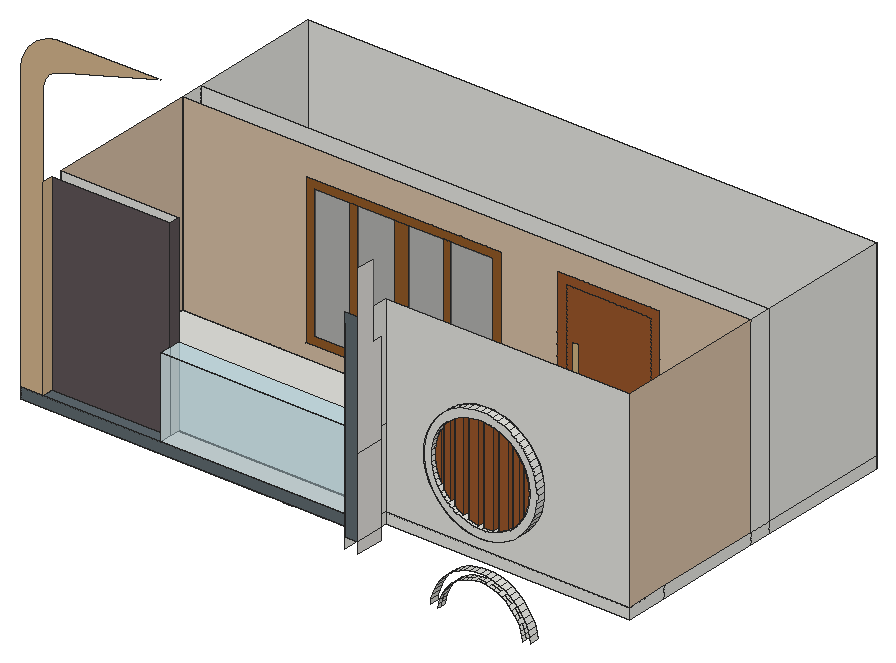
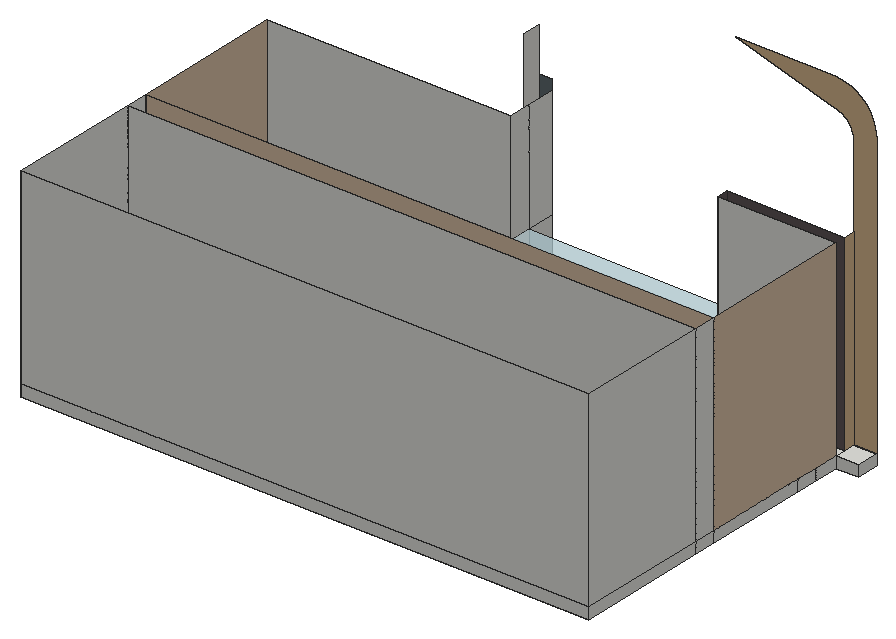
# SketchUp Ruby script. Lengths in inches.
U = 1.inch
M = Sketchup.active_model
def pt(a) = Geom::Point3d.new(a.map { |v| v * U })
def face(e, loops, mat)
  f = e.add_face(loops[0].map { |a| pt(a) })
  loops[1..].each { |l| e.add_face(l.map { |a| pt(a) }).erase! }
  f.material = f.back_material = mat if mat
  f
end
# faces: each face lists its corners as indices into pts; further lists are holes
def faces(e, pts, list, mat = nil) = list.each { |f| face(e, (f[0].is_a?(Array) ? f : [f]).map { |l| l.map { |i| pts[i] } }, mat) }
# xy, xz, yz: faces in a plane at the given z, y or x. An outline is a flat list of corners, or four numbers for a rectangle; further outlines are holes
def ring(l) = l.size == 4 ? [[l[0], l[1]], [l[2], l[1]], [l[2], l[3]], [l[0], l[3]]] : l.each_slice(2).to_a
def flat(e, list, mat, &to3) = list.each { |f| face(e, (f[0].is_a?(Array) ? f : [f]).map { |l| ring(l).map { |u, v| to3.(u, v) } }, mat) }
def xy(e, z, list, mat = nil) = flat(e, list, mat) { |x, y| [x, y, z] }
def xz(e, y, list, mat = nil) = flat(e, list, mat) { |x, z| [x, y, z] }
def yz(e, x, list, mat = nil) = flat(e, list, mat) { |y, z| [x, y, z] }
def lines(e, pts, list) = list.each { |a, b| e.add_line(pt(pts[a]), pt(pts[b])) }
# prism: a flat outline (further loops are holes) pulled along v
def prism(e, loops, v, mat = nil)
  f = face(e, loops, mat); d = Geom::Vector3d.new(v.map { |x| x * U })
  f.pushpull(f.normal.samedirection?(d) ? d.length : -d.length)
end
def box(e, o, s, mat = nil) = prism(e, [[o, [o[0] + s[0], o[1], o[2]], [o[0] + s[0], o[1] + s[1], o[2]], [o[0], o[1] + s[1], o[2]]]], [0, 0, s[2]], mat)
def at(x, y, z, deg = 0) = Geom::Transformation.translation(pt([x, y, z])) * Geom::Transformation.rotation(ORIGIN, Z_AXIS, deg.degrees)
def axes(o, x, y, z) = Geom::Transformation.new([*x, 0, *y, 0, *z, 0, *pt(o).to_a, 1])
def part(name) = M.definitions.add(name)
# library, detail: a bought-in or finely detailed component or shape, given as its bounding box
def library(name, o, s) = part(name).tap { |d| box(d.entities, o, s) }
def detail(e, o, s) = box(e.add_group.entities, o, s)
def put(e, d, t, mat = nil) = e.add_instance(d, t).tap { |i| i.material = mat if mat }
def group(e, t, mat = nil) = e.add_group.tap { |g| g.transformation = t; g.material = mat if mat }.entities
root = M.entities
M.materials.add("[0035_Tan]").color = [210, 180, 140]
M.materials.add("[Asphalt New]").color = [94, 84, 87]
M.materials.add("[Formica Laminate Dark]").color = [50, 53, 60]
M.materials.add("[Formica Laminate Light]").color = [213, 189, 164]
M.materials.add("[Formica Speckled Grey]1").color = [94, 105, 111]
M.materials.add("[Terrazzo Tile Accent]").color = [224, 221, 217]
M.materials.add("[Translucent Glass Gray]").color = [128, 128, 128]
M.materials["[Translucent Glass Gray]"].alpha = 0.5
M.materials.add("[Translucent Glass Safety]").color = [204, 235, 244]
M.materials["[Translucent Glass Safety]"].alpha = 0.5
M.materials.add("[Wood Cherry Original]").color = [152, 86, 42]
M.materials.add("[Wood Floor Light]").color = [204, 176, 127]
M.materials.add("[Wood Floor Parquet]").color = [145, 89, 39]
xy(root,318.5,[[192.74,22.75,199.15,40.6875],[201.68,22.75,208.09,40.6875],[210.74,22.75,217.15,40.6875],[219.8,22.75,226.21,40.6875],[228.49,22.75,234.9,40.6875],
  [237.55,22.75,243.96,40.6875],[246.43,22.75,252.84,40.6875],[255.74,22.75,262.15,40.6875],[264.27,22.75,277.85,40.6875],[264.27,40.6875,277.85,49.71],
  [17.9375,61.15,34.45,78.66],[17.9375,162.27,472.4375,180.28],[17.9375,180.28,472.4375,287.24]])
xy(root,318.5,[[0,22.75,192.74,22.75,192.74,49.71,199.15,49.71,199.15,22.75,201.68,22.75,201.68,49.71,208.09,49.71,208.09,22.75,210.74,22.75,210.74,49.71,217.15,49.71,217.15,22.75,219.8,22.75,219.8,49.71,226.21,49.71,226.21,22.75,228.49,22.75,228.49,49.71,234.9,49.71,234.9,22.75,237.55,22.75,237.55,49.71,243.96,49.71,243.96,22.75,246.43,22.75,246.43,49.71,252.84,49.71,252.84,22.75,255.74,22.75,255.74,49.71,262.15,49.71,262.15,22.75,264.27,22.75,264.27,49.71,277.85,49.71,277.85,40.6875,472.4375,40.6875,472.4375,162.27,17.9375,162.27,17.9375,78.66,34.45,78.66,34.45,61.15,17.9375,61.15,17.9375,40.6875,0,40.6875]],"[Formica Speckled Grey]1")
xy(root,327.375,[[0,22.75,17.9375,40.6875],[112.18,22.75,277.85,40.6875],[17.9375,31.75,112.18,40.6875],[17.9375,40.6875,472.4375,162.27],[17.9375,162.27,472.4375,180.28],
  [17.9375,180.28,472.4375,287.24]])
xy(root,327.375,[[17.9375,22.75,112.18,31.75]],"[Formica Speckled Grey]1")
xy(root,390.5625,[[112.18,22.75,277.85,40.6875]],"[Translucent Glass Safety]")
xz(root,0,[[277.85,327.375,288.19,488.3125]],"[Formica Speckled Grey]1")
xz(root,15.8125,[[[373.3125,352.86,378.06,353.11,382.75,353.85,387.33,355.08,391.77,356.78,396,358.9375,399.98,361.53,403.67,364.51,407.03,367.87,410.02,371.5625,412.61,375.55,414.76,379.78,416.47,384.21,417.7,388.8,418.4375,393.49,418.6875,398.23,418.4375,402.98,417.7,407.67,416.47,412.26,414.76,416.69,412.61,420.92,410.02,424.91,407.03,428.6,403.67,431.95,399.98,434.94,396,437.53,391.77,439.6875,387.33,441.39,382.75,442.62,378.06,443.36,373.3125,443.61,368.57,443.36,363.88,442.62,359.29,441.39,354.86,439.6875,350.625,437.53,346.64,434.94,342.95,431.95,339.59,428.6,336.6,424.91,334.02,420.92,331.86,416.69,330.16,412.26,328.93,407.67,328.1875,402.98,327.9375,398.23,328.1875,393.49,328.93,388.8,330.16,384.21,331.86,379.78,334.02,375.55,336.6,371.5625,339.59,367.87,342.95,364.51,346.64,361.53,350.625,358.9375,354.86,356.78,359.29,355.08,363.88,353.85,368.57,353.11],[373.3125,359.05,369.22,359.26,365.17,359.91,361.2,360.97,357.375,362.4375,353.72,364.3,350.28,366.53,347.09,369.11,344.19,372.01,341.61,375.2,339.375,378.64,337.51,382.3,336.04,386.125,334.98,390.09,334.34,394.14,334.125,398.23,334.34,402.33,334.98,406.38,336.04,410.34,337.51,414.17,339.375,417.83,341.61,421.27,344.19,424.45,347.09,427.36,350.28,429.9375,353.72,432.17,357.375,434.03,361.2,435.5,365.17,436.5625,369.22,437.21,373.3125,437.42,377.41,437.21,381.46,436.5625,385.42,435.5,389.25,434.03,392.9,432.17,396.34,429.9375,399.53,427.36,402.43,424.45,405.01,421.27,407.25,417.83,409.11,414.17,410.58,410.34,411.64,406.38,412.28,402.33,412.5,398.23,412.28,394.14,411.64,390.09,410.58,386.125,409.11,382.3,407.25,378.64,405.01,375.2,402.43,372.01,399.53,369.11,396.34,366.53,392.9,364.3,389.25,362.4375,385.42,360.97,381.46,359.91,377.41,359.26]]])
xz(root,19.125,[[373.3125,359.05,377.41,359.26,381.46,359.91,381.46,436.5625,377.41,437.21,373.3125,437.42],[369.22,359.26,369.22,437.21,365.17,436.5625,361.2,435.5,361.2,360.97,365.17,359.91],[385.42,360.97,389.25,362.4375,392.9,364.3,392.9,432.17,389.25,434.03,385.42,435.5],[357.375,362.4375,357.375,434.03,353.72,432.17,350.28,429.9375,350.28,366.53,353.72,364.3],[396.34,366.53,399.53,369.11,402.43,372.01,402.43,424.45,399.53,427.36,396.34,429.9375],
  [347.09,369.11,347.09,427.36,344.19,424.45,341.61,421.27,341.61,375.2,344.19,372.01],[405.01,375.2,407.25,378.64,409.11,382.3,410.58,386.125,411.64,390.09,412.28,394.14,412.5,398.23,412.28,402.33,411.64,406.38,410.58,410.34,409.11,414.17,407.25,417.83,405.01,421.27],[339.375,378.64,339.375,417.83,337.51,414.17,336.04,410.34,334.98,406.38,334.34,402.33,334.125,398.23,334.34,394.14,334.98,390.09,336.04,386.125,337.51,382.3]],"[Wood Cherry Original]")
xz(root,22.75,[[[373.3125,352.86,368.57,353.11,363.88,353.85,359.29,355.08,354.86,356.78,350.625,358.9375,346.64,361.53,342.95,364.51,339.59,367.87,336.6,371.5625,334.02,375.55,331.86,379.78,330.16,384.21,328.93,388.8,328.1875,393.49,327.9375,398.23,328.1875,402.98,328.93,407.67,330.16,412.26,331.86,416.69,334.02,420.92,336.6,424.91,339.59,428.6,342.95,431.95,346.64,434.94,350.625,437.53,354.86,439.6875,359.29,441.39,363.88,442.62,368.57,443.36,373.3125,443.61,378.06,443.36,382.75,442.62,387.33,441.39,391.77,439.6875,396,437.53,399.98,434.94,403.67,431.95,407.03,428.6,410.02,424.91,412.61,420.92,414.76,416.69,416.47,412.26,417.7,407.67,418.4375,402.98,418.6875,398.23,418.4375,393.49,417.7,388.8,416.47,384.21,414.76,379.78,412.61,375.55,410.02,371.5625,407.03,367.87,403.67,364.51,399.98,361.53,396,358.9375,391.77,356.78,387.33,355.08,382.75,353.85,378.06,353.11],[373.3125,359.05,377.41,359.26,381.46,359.91,385.42,360.97,389.25,362.4375,392.9,364.3,396.34,366.53,399.53,369.11,402.43,372.01,405.01,375.2,407.25,378.64,409.11,382.3,410.58,386.125,411.64,390.09,412.28,394.14,412.5,398.23,412.28,402.33,411.64,406.38,410.58,410.34,409.11,414.17,407.25,417.83,405.01,421.27,402.43,424.45,399.53,427.36,396.34,429.9375,392.9,432.17,389.25,434.03,385.42,435.5,381.46,436.5625,377.41,437.21,373.3125,437.42,369.22,437.21,365.17,436.5625,361.2,435.5,357.375,434.03,353.72,432.17,350.28,429.9375,347.09,427.36,344.19,424.45,341.61,421.27,339.375,417.83,337.51,414.17,336.04,410.34,334.98,406.38,334.34,402.33,334.125,398.23,334.34,394.14,334.98,390.09,336.04,386.125,337.51,382.3,339.375,378.64,341.61,375.2,344.19,372.01,347.09,369.11,350.28,366.53,353.72,364.3,357.375,362.4375,361.2,360.97,365.17,359.91,369.22,359.26]],[373.3125,359.05,373.3125,437.42,377.41,437.21,381.46,436.5625,381.46,359.91,377.41,359.26],[369.22,359.26,365.17,359.91,361.2,360.97,361.2,435.5,365.17,436.5625,369.22,437.21],[385.42,360.97,385.42,435.5,389.25,434.03,392.9,432.17,392.9,364.3,389.25,362.4375],[357.375,362.4375,353.72,364.3,350.28,366.53,350.28,429.9375,353.72,432.17,357.375,434.03],
  [396.34,366.53,396.34,429.9375,399.53,427.36,402.43,424.45,402.43,372.01,399.53,369.11],[347.09,369.11,344.19,372.01,341.61,375.2,341.61,421.27,344.19,424.45,347.09,427.36],[405.01,375.2,405.01,421.27,407.25,417.83,409.11,414.17,410.58,410.34,411.64,406.38,412.28,402.33,412.5,398.23,412.28,394.14,411.64,390.09,410.58,386.125,409.11,382.3,407.25,378.64],[339.375,378.64,337.51,382.3,336.04,386.125,334.98,390.09,334.34,394.14,334.125,398.23,334.34,402.33,334.98,406.38,336.04,410.34,337.51,414.17,339.375,417.83]])
xz(root,22.75,[[0,327.375,17.9375,327.375,17.9375,545.9,18.09,548.21,18.54,550.47,19.28,552.66,20.3,554.73,21.59,556.65,23.11,558.39,24.85,559.91,26.77,561.19,28.84,562.21,31.02,562.96,33.29,563.41,112.18,586.1875,33.45,586.1875,29.09,585.9,24.8,585.05,20.65,583.64,16.73,581.71,13.09,579.27,9.8,576.39,6.91,573.1,4.48,569.46,2.55,565.54,1.14,561.39,0.29,557.1,0,552.73]],"[0035_Tan]")
xz(root,22.75,[[373.3125,359.05,373.3125,437.42,369.22,437.21,369.22,359.26],[381.46,359.91,385.42,360.97,385.42,435.5,381.46,436.5625],[361.2,360.97,361.2,435.5,357.375,434.03,357.375,362.4375],[392.9,364.3,396.34,366.53,396.34,429.9375,392.9,432.17],[350.28,366.53,350.28,429.9375,347.09,427.36,347.09,369.11],
  [402.43,372.01,405.01,375.2,405.01,421.27,402.43,424.45],[341.61,375.2,341.61,421.27,339.375,417.83,339.375,378.64]],"[Formica Laminate Dark]")
xz(root,22.75,[[0,318.5,277.85,327.375]],"[Formica Speckled Grey]1")
xz(root,22.75,[[112.18,327.375,277.85,390.5625]],"[Translucent Glass Safety]")
xz(root,31.75,[[17.9375,327.375,112.18,479.875]],"[Asphalt New]")
xz(root,40.6875,[[0,318.5,17.9375,327.375],[277.85,318.5,472.4375,327.375],[17.9375,327.375,112.18,479.875],[277.85,327.375,472.4375,479.875]])
xz(root,40.6875,[[112.18,327.375,277.85,390.5625]],"[Translucent Glass Safety]")
xz(root,162.27,[[17.9375,318.5,472.4375,327.375]])
xz(root,162.27,[[[17.9375,327.375,317.44,327.375,317.44,460.36,399.63,460.36,399.63,327.375,472.4375,327.375,472.4375,479.875,17.9375,479.875],[116.58,338.54,272.76,458.17]]],"[Formica Laminate Light]")
xz(root,162.27,[[123.45,345.41,151.96,451.3],[158.03,345.41,188.04,451.3],[199.2,345.41,226.47,451.3],[232.54,345.41,265.89,451.3]],"[Translucent Glass Gray]")
xz(root,162.27,[[[317.44,327.375,399.63,460.36],[324.89,334.82,392.1875,452.91]],[[324.89,334.82,392.1875,452.91],[329.4,378.4375,334.59,413.875]]],"[Wood Cherry Original]")
xz(root,162.27,[[329.4,378.4375,334.59,413.875]],"[Wood Floor Light]")
xz(root,162.27,[[[116.58,338.54,272.76,458.17],[123.45,345.41,265.89,451.3]],[151.96,345.41,158.03,451.3],[188.04,345.41,199.2,451.3],[226.47,345.41,232.54,451.3]],"[Wood Floor Parquet]")
xz(root,180.28,[[17.9375,318.5,472.4375,327.375],[17.9375,327.375,472.4375,479.875]])
xz(root,287.24,[[17.9375,318.5,472.4375,327.375],[17.9375,327.375,472.4375,479.875]])
yz(root,0,[[22.75,318.5,40.6875,327.375]])
yz(root,17.9375,[[40.6875,318.5,61.15,327.375],[61.15,318.5,78.66,327.375],[78.66,318.5,162.27,327.375],[162.27,318.5,180.28,327.375],[180.28,318.5,287.24,327.375],
  [162.27,327.375,180.28,479.875],[180.28,327.375,287.24,479.875]])
yz(root,17.9375,[[22.75,327.375,31.75,479.875]],"[0035_Tan]")
yz(root,17.9375,[[40.6875,327.375,162.27,479.875]],"[Formica Laminate Light]")
yz(root,112.18,[[22.75,327.375,31.75,390.5625],[31.75,327.375,40.6875,390.5625]])
yz(root,112.18,[[31.75,390.5625,40.6875,479.875]],"[Asphalt New]")
yz(root,277.85,[[0,318.5,22.75,327.375],[22.75,318.5,40.6875,327.375],[0,327.375,22.75,390.5625],[22.75,327.375,40.6875,390.5625],[0,390.5625,22.75,479.875],
  [22.75,390.5625,40.6875,479.875]])
yz(root,288.19,[[0,318.5,22.75,327.375],[0,327.375,22.75,390.5625],[0,390.5625,22.75,390.5625,22.75,464.44,14.3125,464.44,14.3125,523.3125,0,523.3125]],"[Terrazzo Tile Accent]")
yz(root,339.375,[[19.125,378.64,22.75,417.83]],"[Wood Cherry Original]")
yz(root,341.61,[[19.125,375.2,22.75,421.27]],"[Wood Cherry Original]")
yz(root,347.09,[[19.125,369.11,22.75,427.36]],"[Wood Cherry Original]")
yz(root,350.28,[[19.125,366.53,22.75,429.9375]],"[Wood Cherry Original]")
yz(root,357.375,[[19.125,362.4375,22.75,434.03]],"[Wood Cherry Original]")
yz(root,361.2,[[19.125,360.97,22.75,435.5]],"[Wood Cherry Original]")
yz(root,369.22,[[19.125,359.26,22.75,437.21]],"[Wood Cherry Original]")
yz(root,373.3125,[[19.125,359.05,22.75,437.42]],"[Wood Cherry Original]")
yz(root,381.46,[[19.125,359.91,22.75,436.5625]],"[Wood Cherry Original]")
yz(root,385.42,[[19.125,360.97,22.75,435.5]],"[Wood Cherry Original]")
yz(root,392.9,[[19.125,364.3,22.75,432.17]],"[Wood Cherry Original]")
yz(root,396.34,[[19.125,366.53,22.75,429.9375]],"[Wood Cherry Original]")
yz(root,402.43,[[19.125,372.01,22.75,424.45]],"[Wood Cherry Original]")
yz(root,405.01,[[19.125,375.2,22.75,421.27]],"[Wood Cherry Original]")
yz(root,472.4375,[[40.6875,318.5,75.25,327.375],[75.25,318.5,162.27,327.375],[162.27,318.5,180.28,327.375],[180.28,318.5,287.24,327.375],[162.27,327.375,180.28,479.875],
  [180.28,327.375,287.24,479.875]])
yz(root,472.4375,[[40.6875,327.375,162.27,479.875]],"[Formica Laminate Light]")
p = [[339.47,15.8125,290.96],[339.47,18.4375,290.96],[340.02,18.4375,294.48],[340.02,15.8125,294.48],[406.6,15.8125,294.48],[406.6,18.4375,294.48],
  [407.16,18.4375,290.96],[407.16,15.8125,290.96],[339.47,22.75,290.96],[340.02,22.75,294.48],[406.6,22.75,294.48],[407.16,22.75,290.96],
  [333.97,22.75,295.77],[333.3125,22.75,291.61],[333.3125,15.8125,291.61],[333.97,15.8125,295.77],[413.3125,22.75,291.61],[412.65,22.75,295.77],
  [412.65,15.8125,295.77],[413.3125,15.8125,291.61],[340.95,18.4375,297.92],[340.95,15.8125,297.92],[405.68,15.8125,297.92],[405.68,18.4375,297.92],
  [340.95,22.75,297.92],[405.68,22.75,297.92],[335.06,22.75,299.83],[335.06,15.8125,299.83],[411.5625,22.75,299.83],[411.5625,15.8125,299.83],
  [342.22,18.4375,301.25],[342.22,15.8125,301.25],[404.4,15.8125,301.25],[404.4,18.4375,301.25],[342.22,22.75,301.25],[404.4,22.75,301.25],
  [336.57,22.75,303.76],[336.57,15.8125,303.76],[410.06,22.75,303.76],[410.06,15.8125,303.76],[343.84,22.75,304.42],[343.84,18.4375,304.42],
  [343.84,15.8125,304.42],[402.78,22.75,304.42],[402.78,15.8125,304.42],[402.78,18.4375,304.42],[338.48,22.75,307.52],[338.48,15.8125,307.52],
  [408.14,22.75,307.52],[408.14,15.8125,307.52],[345.78,18.4375,307.41],[345.78,15.8125,307.41],[400.84,15.8125,307.41],[400.84,18.4375,307.41],
  [345.78,22.75,307.41],[400.84,22.75,307.41],[348.02,18.4375,310.18],[348.02,15.8125,310.18],[398.6,15.8125,310.18],[398.6,18.4375,310.18],
  [348.02,22.75,310.18],[398.6,22.75,310.18],[340.77,22.75,311.05],[340.77,15.8125,311.05],[405.85,22.75,311.05],[405.85,15.8125,311.05],
  [350.54,22.75,312.7],[350.54,18.4375,312.7],[350.54,15.8125,312.7],[396.08,22.75,312.7],[396.08,15.8125,312.7],[396.08,18.4375,312.7],
  [343.42,22.75,314.32],[343.42,15.8125,314.32],[403.2,22.75,314.32],[403.2,15.8125,314.32],[353.31,18.4375,314.9375],[353.31,15.8125,314.9375],
  [393.31,15.8125,314.9375],[393.31,18.4375,314.9375],[353.31,22.75,314.9375],[393.31,22.75,314.9375],[346.4,22.75,317.3],[346.4,15.8125,317.3],
  [400.23,22.75,317.3],[400.23,15.8125,317.3],[356.3,18.4375,316.875],[356.3,15.8125,316.875],[390.33,15.8125,316.875],[390.33,18.4375,316.875],
  [356.3,22.75,316.875],[390.33,22.75,316.875],[359.47,22.75,318.49],[359.47,18.4375,318.49],[359.47,15.8125,318.49],[387.15,22.75,318.49],
  [387.15,15.8125,318.49],[387.15,18.4375,318.49],[349.67,22.75,319.94],[349.67,15.8125,319.94],[396.95,22.75,319.94],[396.95,15.8125,319.94],
  [362.8,18.4375,319.77],[362.8,15.8125,319.77],[383.83,15.8125,319.77],[383.83,18.4375,319.77],[362.8,22.75,319.77],[383.83,22.75,319.77],
  [366.24,18.4375,320.69],[366.24,15.8125,320.69],[380.39,15.8125,320.69],[380.39,18.4375,320.69],[366.24,22.75,320.69],[380.39,22.75,320.69],
  [353.2,22.75,322.24],[353.2,15.8125,322.24],[393.42,22.75,322.24],[393.42,15.8125,322.24],[369.75,22.75,321.25],[369.75,18.4375,321.25],
  [369.75,15.8125,321.25],[376.87,22.75,321.25],[376.87,15.8125,321.25],[376.87,18.4375,321.25],[373.3125,18.4375,321.4375],[373.3125,15.8125,321.4375],
  [373.3125,22.75,321.4375],[356.95,22.75,324.15],[356.95,15.8125,324.15],[389.67,22.75,324.15],[389.67,15.8125,324.15],[360.88,22.75,325.66],
  [360.88,15.8125,325.66],[385.74,22.75,325.66],[385.74,15.8125,325.66],[364.95,22.75,326.75],[364.95,15.8125,326.75],[381.67,22.75,326.75],
  [381.67,15.8125,326.75],[369.11,22.75,327.41],[369.11,15.8125,327.41],[377.52,22.75,327.41],[377.52,15.8125,327.41],[373.3125,22.75,327.625],
  [373.3125,15.8125,327.625],[368.57,22.75,353.11],[373.3125,22.75,352.86],[373.3125,15.8125,352.86],[368.57,15.8125,353.11],[378.06,22.75,353.11],
  [378.06,15.8125,353.11],[363.88,22.75,353.85],[363.88,15.8125,353.85],[382.75,22.75,353.85],[382.75,15.8125,353.85],[359.29,22.75,355.08],
  [359.29,15.8125,355.08],[387.33,22.75,355.08],[387.33,15.8125,355.08],[354.86,22.75,356.78],[354.86,15.8125,356.78],[391.77,22.75,356.78],
  [391.77,15.8125,356.78],[350.625,22.75,358.9375],[350.625,15.8125,358.9375],[396,22.75,358.9375],[396,15.8125,358.9375],[346.64,22.75,361.53],
  [346.64,15.8125,361.53],[399.98,22.75,361.53],[399.98,15.8125,361.53],[373.3125,22.75,359.05],[369.22,22.75,359.26],[369.22,19.125,359.26],
  [369.22,15.8125,359.26],[373.3125,15.8125,359.05],[373.3125,19.125,359.05],[377.41,15.8125,359.26],[377.41,19.125,359.26],[377.41,22.75,359.26],
  [365.17,19.125,359.91],[365.17,15.8125,359.91],[381.46,15.8125,359.91],[381.46,19.125,359.91],[365.17,22.75,359.91],[381.46,22.75,359.91],
  [361.2,19.125,360.97],[361.2,15.8125,360.97],[385.42,22.75,360.97],[385.42,15.8125,360.97],[385.42,19.125,360.97],[361.2,22.75,360.97],
  [357.375,22.75,362.4375],[357.375,19.125,362.4375],[357.375,15.8125,362.4375],[389.25,15.8125,362.4375],[389.25,19.125,362.4375],[389.25,22.75,362.4375],
  [342.95,22.75,364.51],[342.95,15.8125,364.51],[403.67,22.75,364.51],[403.67,15.8125,364.51],[353.72,19.125,364.3],[353.72,15.8125,364.3],
  [392.9,15.8125,364.3],[392.9,19.125,364.3],[353.72,22.75,364.3],[392.9,22.75,364.3],[350.28,19.125,366.53],[350.28,15.8125,366.53],
  [396.34,22.75,366.53],[396.34,15.8125,366.53],[396.34,19.125,366.53],[350.28,22.75,366.53],[339.59,22.75,367.87],[339.59,15.8125,367.87],
  [407.03,22.75,367.87],[407.03,15.8125,367.87],[347.09,22.75,369.11],[347.09,19.125,369.11],[347.09,15.8125,369.11],[399.53,15.8125,369.11],
  [399.53,19.125,369.11],[399.53,22.75,369.11],[336.6,22.75,371.5625],[336.6,15.8125,371.5625],[410.02,22.75,371.5625],[410.02,15.8125,371.5625],
  [344.19,19.125,372.01],[344.19,15.8125,372.01],[402.43,15.8125,372.01],[402.43,19.125,372.01],[344.19,22.75,372.01],[402.43,22.75,372.01],
  [334.02,22.75,375.55],[334.02,15.8125,375.55],[412.61,22.75,375.55],[412.61,15.8125,375.55],[341.61,19.125,375.2],[341.61,15.8125,375.2],
  [405.01,22.75,375.2],[405.01,15.8125,375.2],[405.01,19.125,375.2],[341.61,22.75,375.2],[339.375,22.75,378.64],[339.375,19.125,378.64],
  [339.375,15.8125,378.64],[407.25,15.8125,378.64],[407.25,19.125,378.64],[407.25,22.75,378.64],[331.86,22.75,379.78],[331.86,15.8125,379.78],
  [414.76,22.75,379.78],[414.76,15.8125,379.78],[337.51,19.125,382.3],[337.51,15.8125,382.3],[409.11,15.8125,382.3],[409.11,19.125,382.3],
  [337.51,22.75,382.3],[409.11,22.75,382.3],[330.16,22.75,384.21],[330.16,15.8125,384.21],[416.47,22.75,384.21],[416.47,15.8125,384.21],
  [336.04,19.125,386.125],[336.04,15.8125,386.125],[410.58,15.8125,386.125],[410.58,19.125,386.125],[336.04,22.75,386.125],[410.58,22.75,386.125],
  [328.93,22.75,388.8],[328.93,15.8125,388.8],[417.7,22.75,388.8],[417.7,15.8125,388.8],[334.98,19.125,390.09],[334.98,15.8125,390.09],
  [411.64,15.8125,390.09],[411.64,19.125,390.09],[334.98,22.75,390.09],[411.64,22.75,390.09],[328.1875,22.75,393.49],[328.1875,15.8125,393.49],
  [418.4375,22.75,393.49],[418.4375,15.8125,393.49],[334.34,19.125,394.14],[334.34,15.8125,394.14],[412.28,15.8125,394.14],[412.28,19.125,394.14],
  [334.34,22.75,394.14],[412.28,22.75,394.14],[327.9375,22.75,398.23],[327.9375,15.8125,398.23],[418.6875,22.75,398.23],[418.6875,15.8125,398.23],
  [334.125,19.125,398.23],[334.125,15.8125,398.23],[412.5,15.8125,398.23],[412.5,19.125,398.23],[334.125,22.75,398.23],[412.5,22.75,398.23],
  [328.1875,22.75,402.98],[328.1875,15.8125,402.98],[334.34,19.125,402.33],[334.34,15.8125,402.33],[412.28,15.8125,402.33],[412.28,19.125,402.33],
  [418.4375,22.75,402.98],[418.4375,15.8125,402.98],[334.34,22.75,402.33],[412.28,22.75,402.33],[334.98,19.125,406.38],[334.98,15.8125,406.38],
  [411.64,15.8125,406.38],[411.64,19.125,406.38],[334.98,22.75,406.38],[411.64,22.75,406.38],[328.93,22.75,407.67],[328.93,15.8125,407.67],
  [417.7,22.75,407.67],[417.7,15.8125,407.67],[336.04,19.125,410.34],[336.04,15.8125,410.34],[410.58,15.8125,410.34],[410.58,19.125,410.34],
  [336.04,22.75,410.34],[410.58,22.75,410.34],[330.16,22.75,412.26],[330.16,15.8125,412.26],[416.47,22.75,412.26],[416.47,15.8125,412.26],
  [337.51,19.125,414.17],[337.51,15.8125,414.17],[409.11,15.8125,414.17],[409.11,19.125,414.17],[337.51,22.75,414.17],[409.11,22.75,414.17],
  [331.86,22.75,416.69],[331.86,15.8125,416.69],[414.76,22.75,416.69],[414.76,15.8125,416.69],[339.375,19.125,417.83],[339.375,15.8125,417.83],
  [407.25,15.8125,417.83],[407.25,19.125,417.83],[339.375,22.75,417.83],[407.25,22.75,417.83],[334.02,22.75,420.92],[334.02,15.8125,420.92],
  [412.61,22.75,420.92],[412.61,15.8125,420.92],[341.61,22.75,421.27],[341.61,19.125,421.27],[341.61,15.8125,421.27],[405.01,15.8125,421.27],
  [405.01,19.125,421.27],[405.01,22.75,421.27],[336.6,22.75,424.91],[336.6,15.8125,424.91],[410.02,22.75,424.91],[410.02,15.8125,424.91],
  [344.19,19.125,424.45],[344.19,15.8125,424.45],[402.43,22.75,424.45],[402.43,15.8125,424.45],[402.43,19.125,424.45],[344.19,22.75,424.45],
  [347.09,19.125,427.36],[347.09,15.8125,427.36],[399.53,15.8125,427.36],[399.53,19.125,427.36],[347.09,22.75,427.36],[399.53,22.75,427.36],
  [339.59,22.75,428.6],[339.59,15.8125,428.6],[407.03,22.75,428.6],[407.03,15.8125,428.6],[350.28,22.75,429.9375],[350.28,19.125,429.9375],
  [350.28,15.8125,429.9375],[396.34,15.8125,429.9375],[396.34,19.125,429.9375],[396.34,22.75,429.9375],[342.95,22.75,431.95],[342.95,15.8125,431.95],
  [403.67,22.75,431.95],[403.67,15.8125,431.95],[353.72,19.125,432.17],[353.72,15.8125,432.17],[392.9,22.75,432.17],[392.9,15.8125,432.17],
  [392.9,19.125,432.17],[353.72,22.75,432.17],[346.64,22.75,434.94],[346.64,15.8125,434.94],[399.98,22.75,434.94],[399.98,15.8125,434.94],
  [357.375,19.125,434.03],[357.375,15.8125,434.03],[389.25,15.8125,434.03],[389.25,19.125,434.03],[357.375,22.75,434.03],[389.25,22.75,434.03],
  [361.2,22.75,435.5],[361.2,19.125,435.5],[361.2,15.8125,435.5],[385.42,15.8125,435.5],[385.42,19.125,435.5],[385.42,22.75,435.5],
  [350.625,22.75,437.53],[350.625,15.8125,437.53],[396,22.75,437.53],[396,15.8125,437.53],[365.17,19.125,436.5625],[365.17,15.8125,436.5625],
  [381.46,22.75,436.5625],[381.46,15.8125,436.5625],[381.46,19.125,436.5625],[365.17,22.75,436.5625],[369.22,19.125,437.21],[369.22,15.8125,437.21],
  [377.41,15.8125,437.21],[377.41,19.125,437.21],[369.22,22.75,437.21],[377.41,22.75,437.21],[373.3125,22.75,437.42],[373.3125,19.125,437.42],
  [373.3125,15.8125,437.42],[354.86,22.75,439.6875],[354.86,15.8125,439.6875],[391.77,22.75,439.6875],[391.77,15.8125,439.6875],[359.29,22.75,441.39],
  [359.29,15.8125,441.39],[387.33,22.75,441.39],[387.33,15.8125,441.39],[363.88,22.75,442.62],[363.88,15.8125,442.62],[382.75,22.75,442.62],
  [382.75,15.8125,442.62],[368.57,22.75,443.36],[368.57,15.8125,443.36],[378.06,22.75,443.36],[378.06,15.8125,443.36],[373.3125,22.75,443.61],
  [373.3125,15.8125,443.61]]
faces(root,p,[[0,1,2,3],[4,5,6,7],[8,9,2,1],[10,11,6,5],[12,13,14,15],[16,17,18,19],[3,2,20,21],[22,23,5,4],
  [9,24,20,2],[25,10,5,23],[26,12,15,27],[17,28,29,18],[21,20,30,31],[32,33,23,22],[24,34,30,20],[35,25,23,33],
  [36,26,27,37],[28,38,39,29],[34,40,41,42,31,30],[43,35,33,32,44,45],[46,36,37,47],[38,48,49,39],[42,41,50,51],[52,53,45,44],
  [40,54,50,41],[55,43,45,53],[51,50,56,57],[58,59,53,52],[54,60,56,50],[61,55,53,59],[62,46,47,63],[48,64,65,49],
  [60,66,67,68,57,56],[69,61,59,58,70,71],[72,62,63,73],[64,74,75,65],[68,67,76,77],[78,79,71,70],[66,80,76,67],[81,69,71,79],
  [82,72,73,83],[74,84,85,75],[77,76,86,87],[88,89,79,78],[80,90,86,76],[91,81,79,89],[90,92,93,94,87,86],[95,91,89,88,96,97],
  [98,82,83,99],[84,100,101,85],[94,93,102,103],[104,105,97,96],[92,106,102,93],[107,95,97,105],[103,102,108,109],[110,111,105,104],
  [106,112,108,102],[113,107,105,111],[114,98,99,115],[100,116,117,101],[112,118,119,120,109,108],[121,113,111,110,122,123],[120,119,124,125],[125,124,123,122],
  [118,126,124,119],[126,121,123,124],[127,114,115,128],[116,129,130,117],[131,127,128,132],[129,133,134,130],[135,131,132,136],[133,137,138,134],
  [139,135,136,140],[137,141,142,138],[143,139,140,144],[141,143,144,142],[145,146,147,148],[146,149,150,147],[151,145,148,152],[149,153,154,150],
  [155,151,152,156],[153,157,158,154],[159,155,156,160],[157,161,162,158],[163,159,160,164],[161,165,166,162],[167,163,164,168],[165,169,170,166],
  [171,172,173,174,175,176],[177,178,176,175],[179,171,176,178],[174,173,180,181],[182,183,178,177],[172,184,180,173],[185,179,178,183],[181,180,186,187],
  [188,185,183,182,189,190],[184,191,186,180],[191,192,193,194,187,186],[195,196,190,189],[197,188,190,196],[198,167,168,199],[169,200,201,170],[194,193,202,203],
  [204,205,196,195],[192,206,202,193],[207,197,196,205],[203,202,208,209],[210,207,205,204,211,212],[206,213,208,202],[214,198,199,215],[200,216,217,201],
  [213,218,219,220,209,208],[221,222,212,211],[223,210,212,222],[224,214,215,225],[216,226,227,217],[220,219,228,229],[230,231,222,221],[218,232,228,219],
  [233,223,222,231],[234,224,225,235],[226,236,237,227],[229,228,238,239],[240,233,231,230,241,242],[232,243,238,228],[243,244,245,246,239,238],[247,248,242,241],
  [249,240,242,248],[250,234,235,251],[236,252,253,237],[246,245,254,255],[256,257,248,247],[244,258,254,245],[259,249,248,257],[260,250,251,261],
  [252,262,263,253],[255,254,264,265],[266,267,257,256],[258,268,264,254],[269,259,257,267],[270,260,261,271],[262,272,273,263],[265,264,274,275],
  [276,277,267,266],[268,278,274,264],[279,269,267,277],[280,270,271,281],[272,282,283,273],[275,274,284,285],[286,287,277,276],[278,288,284,274],
  [289,279,277,287],[290,280,281,291],[282,292,293,283],[285,284,294,295],[296,297,287,286],[288,298,294,284],[299,289,287,297],[300,290,291,301],
  [295,294,302,303],[304,305,297,296],[292,306,307,293],[298,308,302,294],[309,299,297,305],[303,302,310,311],[312,313,305,304],[308,314,310,302],
  [315,309,305,313],[316,300,301,317],[306,318,319,307],[311,310,320,321],[322,323,313,312],[314,324,320,310],[325,315,313,323],[326,316,317,327],
  [318,328,329,319],[321,320,330,331],[332,333,323,322],[324,334,330,320],[335,325,323,333],[336,326,327,337],[328,338,339,329],[331,330,340,341],
  [342,343,333,332],[334,344,340,330],[345,335,333,343],[346,336,337,347],[338,348,349,339],[344,350,351,352,341,340],[353,354,343,342],[355,345,343,354],
  [356,346,347,357],[348,358,359,349],[352,351,360,361],[362,355,354,353,363,364],[350,365,360,351],[361,360,366,367],[368,369,364,363],[365,370,366,360],
  [371,362,364,369],[372,356,357,373],[358,374,375,359],[370,376,377,378,367,366],[379,380,369,368],[381,371,369,380],[382,372,373,383],[374,384,385,375],
  [378,377,386,387],[388,381,380,379,389,390],[376,391,386,377],[392,382,383,393],[384,394,395,385],[387,386,396,397],[398,399,390,389],[391,400,396,386],
  [401,388,390,399],[400,402,403,404,397,396],[405,406,399,398],[407,401,399,406],[408,392,393,409],[394,410,411,395],[404,403,412,413],[414,407,406,405,415,416],
  [402,417,412,403],[413,412,418,419],[420,421,416,415],[417,422,418,412],[423,414,416,421],[422,424,425,426,419,418],[426,425,421,420],[424,423,421,425],
  [427,408,409,428],[410,429,430,411],[431,427,428,432],[429,433,434,430],[435,431,432,436],[433,437,438,434],[439,435,436,440],[437,441,442,438],
  [443,439,440,444],[441,443,444,442]])
